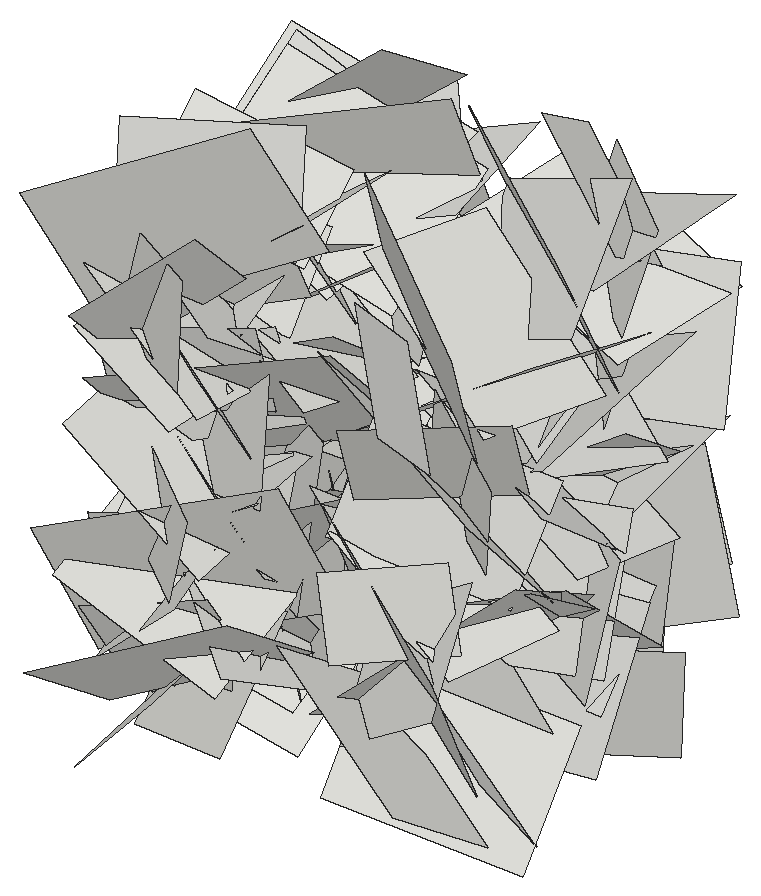
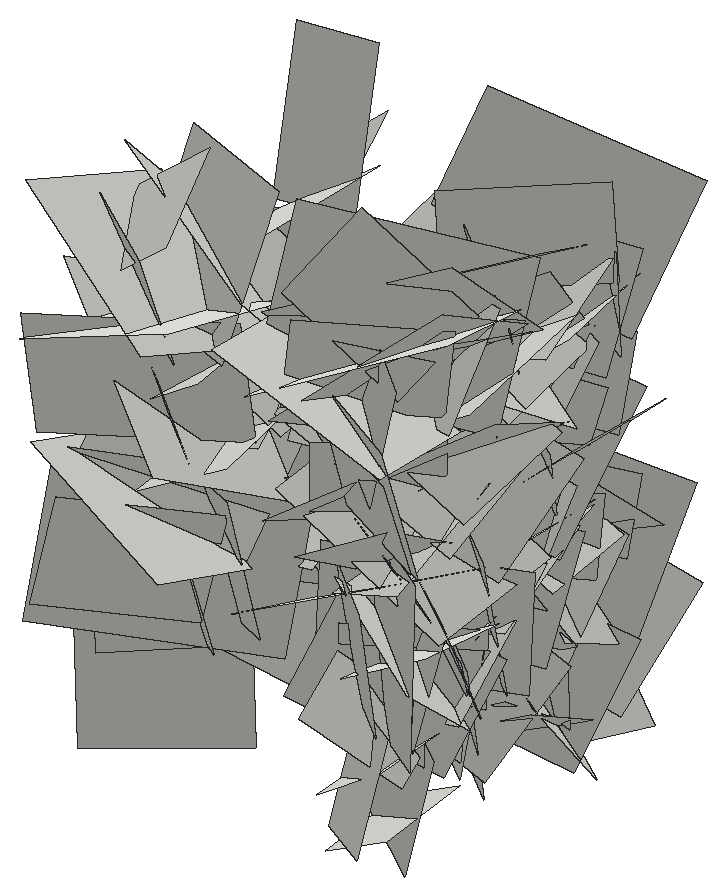
# SketchUp Ruby script. Lengths in inches.
U = 1.inch
M = Sketchup.active_model
def pt(a) = Geom::Point3d.new(a.map { |v| v * U })
def face(e, loops, mat)
  f = e.add_face(loops[0].map { |a| pt(a) })
  loops[1..].each { |l| e.add_face(l.map { |a| pt(a) }).erase! }
  f.material = f.back_material = mat if mat
  f
end
# faces: each face lists its corners as indices into pts; further lists are holes
def faces(e, pts, list, mat = nil) = list.each { |f| face(e, (f[0].is_a?(Array) ? f : [f]).map { |l| l.map { |i| pts[i] } }, mat) }
# xy, xz, yz: faces in a plane at the given z, y or x. An outline is a flat list of corners, or four numbers for a rectangle; further outlines are holes
def ring(l) = l.size == 4 ? [[l[0], l[1]], [l[2], l[1]], [l[2], l[3]], [l[0], l[3]]] : l.each_slice(2).to_a
def flat(e, list, mat, &to3) = list.each { |f| face(e, (f[0].is_a?(Array) ? f : [f]).map { |l| ring(l).map { |u, v| to3.(u, v) } }, mat) }
def xy(e, z, list, mat = nil) = flat(e, list, mat) { |x, y| [x, y, z] }
def xz(e, y, list, mat = nil) = flat(e, list, mat) { |x, z| [x, y, z] }
def yz(e, x, list, mat = nil) = flat(e, list, mat) { |y, z| [x, y, z] }
def lines(e, pts, list) = list.each { |a, b| e.add_line(pt(pts[a]), pt(pts[b])) }
# prism: a flat outline (further loops are holes) pulled along v
def prism(e, loops, v, mat = nil)
  f = face(e, loops, mat); d = Geom::Vector3d.new(v.map { |x| x * U })
  f.pushpull(f.normal.samedirection?(d) ? d.length : -d.length)
end
def box(e, o, s, mat = nil) = prism(e, [[o, [o[0] + s[0], o[1], o[2]], [o[0] + s[0], o[1] + s[1], o[2]], [o[0], o[1] + s[1], o[2]]]], [0, 0, s[2]], mat)
def at(x, y, z, deg = 0) = Geom::Transformation.translation(pt([x, y, z])) * Geom::Transformation.rotation(ORIGIN, Z_AXIS, deg.degrees)
def axes(o, x, y, z) = Geom::Transformation.new([*x, 0, *y, 0, *z, 0, *pt(o).to_a, 1])
def part(name) = M.definitions.add(name)
# library, detail: a bought-in or finely detailed component or shape, given as its bounding box
def library(name, o, s) = part(name).tap { |d| box(d.entities, o, s) }
def detail(e, o, s) = box(e.add_group.entities, o, s)
def put(e, d, t, mat = nil) = e.add_instance(d, t).tap { |i| i.material = mat if mat }
def group(e, t, mat = nil) = e.add_group.tap { |g| g.transformation = t; g.material = mat if mat }.entities
root = M.entities
c1 = part("Component\#6")
p = [[0.01,0,0],[0,3.24,4.54],[4.32,3.24,4.54],[4.33,0,0]]
faces(c1.entities,p,[[0,1,2,3]])
put(root,c1,axes([28.31,153.18,27.99],[0.08911,-1.01671,-0.11332],[0.1646,-0.0997,1.00972],[-1.07181,-0.09984,0.14565]))
put(root,c1,axes([24.34,160.42,26.72],[-0.04031,-0.6417,-0.5437],[0.04231,-0.54502,0.64047],[0.89052,-0.00315,-0.05504]))
put(root,c1,axes([28.31,152.86,32.22],[0.07765,-0.95123,0.12327],[0.10469,0.13045,0.94796],[-1.01133,-0.05954,0.1076]))
put(root,c1,axes([28.31,152.23,36.27],[-0.17612,0.33723,0.58016],[0.03508,0.60107,-0.33991],[-0.71045,-0.05392,-0.16061]))
put(root,c1,axes([24.34,156.02,27.27],[0.01737,0.78195,0.05447],[0.0729,0.05284,-0.77921],[0.82768,-0.02106,0.06749]))
put(root,c1,axes([24.34,151.43,29.49],[-0.01376,0.93036,0.01045],[-0.09599,0.00914,-0.92605],[0.98156,0.01394,-0.09041]))
put(root,c1,axes([24.34,155.63,34.51],[-0.04715,-0.7148,-0.47013],[0.06325,-0.47221,0.71232],[0.90467,-0.00424,-0.0743]))
put(root,c1,axes([28.31,159.35,19.53],[-0.12506,-0.65018,0.20227],[0.00025,0.20525,0.65988],[-0.72178,0.11273,-0.03482]))
put(root,c1,axes([28.31,154.14,39.875],[0.07687,-0.17009,-0.90128],[0.07958,-0.89996,0.17589],[-0.96896,-0.0874,-0.05706]))
put(root,c1,axes([24.34,161.57,34.4],[-0.05292,-0.24359,-0.78611],[0.1523,-0.77804,0.23197],[0.85897,0.12294,-0.08956]))
put(root,c1,axes([24.34,150.44,37.52],[-0.01758,-0.03984,-0.83316],[0.08726,-0.82933,0.03802],[0.87984,0.08145,-0.02042]))
put(root,c1,axes([24.34,152.86,25.21],[0.07237,-0.84668,-0.40971],[-0.16913,-0.41526,0.83156],[0.98259,-0.00911,0.17331]))
put(root,c1,axes([24.34,151.53,22],[-0.08087,0.78957,0.40941],[0.10212,0.41583,-0.78401],[0.93722,0.02282,0.12075]))
put(root,c1,axes([24.34,158.82,28.52],[-0.0834,-0.34729,-0.88838],[0.00654,-0.89156,0.34799],[1.01106,-0.02288,-0.07553]))
put(root,c1,axes([28.31,156.05,22.34],[-0.04217,-0.56806,-0.37659],[-0.07293,-0.37196,0.56834],[-0.71876,0.07107,-0.03557]))
put(root,c1,axes([28.31,160.84,30.26],[-0.09118,-0.56201,-0.30691],[-0.0596,-0.30185,0.56849],[-0.67615,0.1024,-0.00872]))
put(root,c1,axes([24.34,154.61,36.92],[-0.07328,1.03426,0.55463],[-0.26621,0.52968,-1.01904],[1.21518,0.17841,-0.1898]))
put(root,c1,axes([28.31,159.76,21.63],[-0.09665,-0.666,0.12875],[0.03078,0.12595,0.67212],[-0.71837,0.095,0.01147]))
put(root,c1,axes([28.31,147.16,24.1],[0.03025,0.92414,0.23442],[0.23339,0.2218,-0.90118],[-0.98329,0.08108,-0.20669]))
put(root,c1,axes([24.34,157.73,31.39],[-0.13129,-0.92283,0.37392],[0.04334,0.37177,0.93107],[1.05456,-0.13017,0.00829]))
put(root,c1,axes([28.31,159.1875,20.3125],[0.01409,-0.35632,0.80543],[0.16766,0.79339,0.34838],[-0.91839,0.13938,0.07596]))
put(root,c1,axes([28.31,153.92,21.15],[0.0271,-0.2919,0.8704],[0.20523,0.85287,0.28034],[-0.95124,0.17569,0.08528]))
put(root,c1,axes([28.31,149.63,26.39],[0.05575,0.3601,-0.58557],[-0.15834,-0.56726,-0.36226],[-0.71127,0.15451,0.03475]))
put(root,c1,axes([28.31,150.69,21.46],[0.08617,-0.06424,0.73191],[-0.1147,0.7273,0.07585],[-0.77031,-0.11548,0.07058]))
put(root,c1,axes([24.34,152.31,24.83],[0.14132,0.38772,0.61473],[0.11706,0.60692,-0.40674],[0.76145,-0.16526,-0.05156]))
put(root,c1,axes([24.34,150.4,30.92],[0.04252,-0.27759,0.76161],[0.13298,0.75548,0.26875],[0.84891,-0.10444,-0.08025]))
put(root,c1,axes([28.31,156.49,28.09],[-0.01227,0.36562,0.53928],[-0.0952,0.53332,-0.36351],[-0.68404,-0.08079,0.04092]))
put(root,c1,axes([24.34,150.56,37.37],[0.01495,0.72639,-0.4873],[0.06872,-0.48689,-0.7239],[0.92463,0.02444,0.06168]))
put(root,c1,axes([28.31,156.34,37.48],[0.20366,-0.78098,-0.33642],[-0.07649,-0.35863,0.79133],[-0.89812,-0.14656,-0.14368]))
put(root,c1,axes([24.34,156.72,22.08],[-0.00521,-0.94479,0.50901],[-0.17637,0.50353,0.93301],[1.12382,0.07464,0.14878]))
put(root,c1,axes([28.31,158.75,26.14],[-0.12859,0.59437,-0.23179],[0.06253,-0.22448,-0.60651],[-0.67335,-0.13435,-0.01206]))
put(root,c1,axes([24.34,154.45,36.57],[0.07713,0.81709,0.22722],[0.03645,0.22503,-0.82021],[0.89825,-0.07929,0.01378]))
put(root,c1,axes([28.31,149.71,29.1],[-0.04042,0.22115,-0.567],[-0.10046,-0.56334,-0.21335],[-0.63725,0.07479,0.0696]))
put(root,c1,axes([28.31,153.82,25.23],[-0.04726,-0.11023,0.59197],[-0.093,0.58845,0.10297],[-0.63147,-0.07841,-0.05947]))
put(root,c1,axes([24.34,150.92,33.45],[-0.01124,-0.40239,0.85237],[0.02564,0.85203,0.40253],[0.99881,-0.0264,-0.00074]))
put(root,c1,axes([24.34,152.27,30.34],[0.04267,0.47891,-0.74389],[0.05776,-0.74459,-0.47642],[0.93603,0.02411,0.06331]))
put(root,c1,axes([24.34,153.79,24.7],[-0.00565,-0.43188,0.90191],[-0.04751,0.90112,0.43124],[1.05892,0.03812,0.02416]))
put(root,c1,axes([24.34,160.9375,37.33],[0.13153,0.12633,-0.90974],[-0.10231,-0.91113,-0.13969],[0.96819,-0.11344,0.10882]))
put(root,c1,axes([28.31,155.3,36.05],[0.02231,-0.46484,-0.62566],[0.10069,-0.6197,0.4636],[-0.82005,-0.08874,0.0399]))
put(root,c1,axes([24.34,155.99,38.05],[0.0315,0.52335,-0.79271],[-0.01447,-0.79278,-0.52391],[1.00678,-0.02777,0.01727]))
put(root,c1,axes([28.31,150.81,32.67],[0.03105,-0.70657,0.01303],[-0.00041,0.01303,0.70717],[-0.74909,-0.02929,0.00015]))
put(root,c1,axes([24.34,158.65,23.12],[-0.03,-0.65446,0.65644],[0.11713,0.64968,0.65248],[0.97555,-0.09812,-0.05816]))
put(root,c1,axes([28.31,151.89,27.92],[-0.07457,-0.37507,-0.49968],[0.035,-0.50437,0.37394],[-0.66135,0.0156,0.07613]))
put(root,c1,axes([28.31,158.01,30.39],[-0.08038,-0.60995,0.00551],[0.02253,0.00291,0.6143],[-0.64618,0.07598,0.02073]))
put(root,c1,axes([28.31,153.52,29.46],[0.08102,0.00764,-0.81457],[0.10707,-0.81193,0.00187],[-0.85682,-0.10074,-0.07679]))
put(root,c1,axes([24.34,152.65,32.7],[-0.31384,1.21799,0.62272],[-0.13011,0.61092,-1.25326],[1.44417,0.31973,0.02242]))
put(root,c1,axes([24.34,149.65,34.23],[-0.2234,-0.54463,1.08834],[-0.02633,1.10624,0.54877],[1.28976,-0.07175,0.19972]))
put(root,c1,axes([28.31,152.7,33.94],[0.15183,0.13661,-0.74127],[-0.04087,-0.75222,-0.14607],[-0.79793,0.06452,-0.13357]))
put(root,c1,axes([28.31,158.73,27.09],[0.13155,-0.14233,-0.74779],[0.00006,-0.75766,0.14422],[-0.80689,-0.02326,-0.12191]))
put(root,c1,axes([24.34,158.66,27.8],[0.19419,0.10037,-0.91545],[-0.10975,-0.92523,-0.12216],[0.97001,-0.12478,0.16945]))
put(root,c1,axes([28.31,156.65,23.33],[-0.01341,0.01203,0.69899],[0.10657,0.69187,-0.01009],[-0.73333,0.10033,-0.01425]))
put(root,c1,axes([24.34,154.96,37.56],[-0.27688,1.1515,0.31839],[0.11464,0.34737,-1.16756],[1.26119,0.22122,0.17603]))
put(root,c1,axes([24.34,152.42,20.54],[-0.05004,-0.6691,0.77955],[0.05919,0.77755,0.67076],[1.08735,-0.07312,-0.00064]))
put(root,c1,axes([28.31,161,38.46],[0.19651,-0.13504,-0.81499],[0.03185,-0.8336,0.14496],[-0.87508,-0.06067,-0.17773]))
put(root,c1,axes([24.34,159.15,23.91],[0.14407,0.13595,-0.90237],[-0.02833,-0.91134,-0.14133],[0.9669,-0.04696,0.13032]))
put(root,c1,axes([24.34,151.25,34.8],[0.16779,0.3958,-0.75565],[0.05631,-0.77163,-0.39305],[0.90246,-0.02545,0.16502]))
put(root,c1,axes([28.31,158.03,24.73],[0.19324,-0.05037,0.89121],[0.15909,0.89838,0.02008],[-0.93272,0.1428,0.18806]))
put(root,c1,axes([24.34,154.4,23.625],[-0.0407,-0.65785,-0.83395],[0.03781,-0.83482,0.65689],[1.12528,0.00426,-0.05223]))
put(root,c1,axes([28.31,157.59,40.82],[0.16311,0.68993,-0.43022],[0.09586,-0.44966,-0.68876],[-0.85651,0.08106,-0.15901]))
put(root,c1,axes([24.34,154.59,24.16],[-0.1724,0.15274,1.09758],[0.17194,1.10067,-0.12914],[1.16199,-0.14021,0.18195]))
put(root,c1,axes([24.34,152.14,28.92],[0.00837,0.82237,-0.50147],[0.16225,-0.49618,-0.8113],[1.00803,0.07304,0.13474]))
put(root,c1,axes([28.31,149.08,38.35],[-0.0057,0.54335,-0.52891],[0.23788,-0.50408,-0.52014],[-0.76776,-0.16022,-0.15723]))
put(root,c1,axes([28.31,157.4,31.875],[0.05779,-0.51798,-0.36432],[0.0587,-0.36037,0.52065],[-0.6687,-0.0764,0.01422]))
put(root,c1,axes([24.34,156.45,32.24],[0.14884,0.843,-0.57449],[-0.06248,-0.57223,-0.85409],[1.07954,-0.14935,0.02978]))
put(root,c1,axes([28.31,160.09,33.87],[0.13785,-0.16653,-0.67513],[0.04892,-0.68326,0.17743],[-0.73546,-0.07666,-0.11474]))
put(root,c1,axes([24.34,156.02,28.65],[-0.0619,-0.85924,0.62732],[0.17366,0.61351,0.85557],[1.11425,-0.14335,-0.09849]))
put(root,c1,axes([28.31,147.9,27.03],[0.12769,0.03013,0.63893],[0.01482,0.64988,-0.03329],[-0.67785,0.01989,0.11963]))
put(root,c1,axes([24.34,156.69,29.48],[-0.02364,1.01192,0.31394],[0.16386,0.31376,-1.00035],[1.11105,-0.02474,0.15421]))
put(root,c1,axes([24.34,161.68,35.57],[-0.09547,-0.29138,-1.10436],[0.14499,-1.10257,0.27976],[1.20197,0.10985,-0.12146]))
put(root,c1,axes([24.34,147.58,26.68],[0.22766,0.71104,0.67114],[-0.02672,0.69094,-0.72395],[1.03608,-0.13842,-0.16614]))
put(root,c1,axes([24.34,153.43,27.14],[0.15407,-0.97446,-0.01303],[0.08051,-0.00181,0.98239],[1.02988,0.14592,-0.07485]))
put(root,c1,axes([24.34,158.93,27.77],[-0.0679,-1.16178,0.21088],[0.08573,0.20637,1.16154],[1.24867,-0.07734,-0.06828]))
put(root,c1,axes([24.34,160.05,30.35],[-0.12426,0.20575,-1.35522],[-0.11745,-1.35714,-0.19646],[1.44825,-0.0924,-0.13221]))
put(root,c1,axes([24.34,157.84,26.69],[0.16666,-0.37984,-0.88441],[0.10341,-0.88523,0.39754],[1.01503,0.15255,0.10471]))
put(root,c1,axes([24.34,153.58,31.99],[0.17505,-0.32324,-0.90395],[0.10086,-0.9072,0.34179],[1.0126,0.14624,0.12223]))
put(root,c1,axes([24.34,151.45,29.33],[0.11063,1.17252,-0.59491],[-0.28501,-0.56514,-1.16101],[1.36425,-0.21315,-0.19431]))
put(root,c1,axes([24.34,155.57,33.875],[0.13701,-1.11756,0.11199],[-0.07264,0.10468,1.12363],[1.18833,0.13525,0.05577]))
put(root,c1,axes([24.34,156.79,29.67],[0.01777,-0.29003,-1.18393],[-0.05362,-1.18318,0.28913],[1.29096,-0.04516,0.0283]))
put(root,c1,axes([24.34,158.37,30.5],[0.12568,-1.12455,0.31778],[-0.06348,0.31314,1.13049],[1.23707,0.13032,0.02572]))
put(root,c1,axes([24.34,152.25,36.24],[-0.0137,1.21221,-0.26433],[0.01965,-0.26413,-1.21218],[1.31499,0.01657,0.01536]))
put(root,c1,axes([24.34,150.2,21.48],[0.03659,-0.96074,0.6365],[0.08804,0.6372,0.9573],[1.21843,-0.01719,-0.08829]))
put(root,c1,axes([24.34,149.67,23.37],[-0.09539,-0.59855,1.14231],[0.08783,1.14003,0.60389],[1.36418,-0.11525,0.041]))
put(root,c1,axes([24.34,153.92,36.42],[0.14295,0.82362,0.79821],[0.11339,0.79118,-0.83443],[1.21047,-0.17138,-0.0161]))
put(root,c1,axes([24.34,156.14,33.68],[0.06217,-0.55405,1.15944],[0.03014,1.16092,0.55332],[1.36179,-0.0004,-0.06518]))
put(root,c1,axes([24.34,157.5625,26.25],[0.15158,-0.38022,-1.22414],[-0.0526,-1.23246,0.37701],[1.35773,-0.0053,0.15127]))
put(root,c1,axes([24.34,161.74,34.71],[0.1652,-1.10091,-0.16395],[0.26327,-0.12698,1.08875],[1.15009,0.1872,-0.22568]))
put(root,c1,axes([24.34,153.73,28.3],[-0.01858,0.99462,-0.84655],[0.29457,-0.8244,-0.97435],[1.35277,0.19318,0.20054]))
put(root,c1,axes([24.34,153.125,28.17],[-0.03085,-0.9293,0.97672],[0.26234,0.95667,0.91759],[1.40479,-0.19906,-0.14991]))
put(root,c1,axes([24.34,153.14,23.91],[0.18,-1.08552,0.79109],[0.08355,0.80406,1.08641],[1.42134,0.0902,-0.16405]))
put(root,c1,axes([38.11,153.14,23.91],[-0.18,-1.08552,0.79109],[-0.08355,0.80406,1.08641],[-1.42134,0.0902,-0.16405]))
put(root,c1,axes([38.11,153.125,28.17],[0.03085,-0.9293,0.97672],[-0.26234,0.95667,0.91759],[-1.40479,-0.19906,-0.14991]))
put(root,c1,axes([38.11,153.73,28.3],[0.01858,0.99462,-0.84655],[-0.29457,-0.8244,-0.97435],[-1.35277,0.19318,0.20054]))
put(root,c1,axes([38.11,161.74,34.71],[-0.1652,-1.10091,-0.16395],[-0.26327,-0.12698,1.08875],[-1.15009,0.1872,-0.22568]))
put(root,c1,axes([38.11,157.5625,26.25],[-0.15158,-0.38022,-1.22414],[0.0526,-1.23246,0.37701],[-1.35773,-0.0053,0.15127]))
put(root,c1,axes([38.11,156.14,33.68],[-0.06217,-0.55405,1.15944],[-0.03014,1.16092,0.55332],[-1.36179,-0.0004,-0.06518]))
put(root,c1,axes([38.11,153.92,36.42],[-0.14295,0.82362,0.79821],[-0.11339,0.79118,-0.83443],[-1.21047,-0.17138,-0.0161]))
put(root,c1,axes([38.11,149.67,23.37],[0.09539,-0.59855,1.14231],[-0.08783,1.14003,0.60389],[-1.36418,-0.11525,0.041]))
put(root,c1,axes([38.11,150.2,21.48],[-0.03659,-0.96074,0.6365],[-0.08804,0.6372,0.9573],[-1.21843,-0.01719,-0.08829]))
put(root,c1,axes([38.11,152.25,36.24],[0.0137,1.21221,-0.26433],[-0.01965,-0.26413,-1.21218],[-1.31499,0.01657,0.01536]))
put(root,c1,axes([38.11,158.37,30.5],[-0.12568,-1.12455,0.31778],[0.06348,0.31314,1.13049],[-1.23707,0.13032,0.02572]))
put(root,c1,axes([38.11,156.79,29.67],[-0.01777,-0.29003,-1.18393],[0.05362,-1.18318,0.28913],[-1.29096,-0.04516,0.0283]))
put(root,c1,axes([38.11,155.57,33.875],[-0.13701,-1.11756,0.11199],[0.07264,0.10468,1.12363],[-1.18833,0.13525,0.05577]))
put(root,c1,axes([38.11,151.45,29.33],[-0.11063,1.17252,-0.59491],[0.28501,-0.56514,-1.16101],[-1.36425,-0.21315,-0.19431]))
put(root,c1,axes([38.11,153.58,31.99],[-0.17505,-0.32324,-0.90395],[-0.10086,-0.9072,0.34179],[-1.0126,0.14624,0.12223]))
put(root,c1,axes([38.11,157.84,26.69],[-0.16666,-0.37984,-0.88441],[-0.10341,-0.88523,0.39754],[-1.01503,0.15255,0.10471]))
put(root,c1,axes([38.11,160.05,30.35],[0.12426,0.20575,-1.35522],[0.11745,-1.35714,-0.19646],[-1.44825,-0.0924,-0.13221]))
put(root,c1,axes([38.11,158.93,27.77],[0.0679,-1.16178,0.21088],[-0.08573,0.20637,1.16154],[-1.24867,-0.07734,-0.06828]))
put(root,c1,axes([38.11,153.43,27.14],[-0.15407,-0.97446,-0.01303],[-0.08051,-0.00181,0.98239],[-1.02988,0.14592,-0.07485]))
put(root,c1,axes([38.11,147.58,26.68],[-0.22766,0.71104,0.67114],[0.02672,0.69094,-0.72395],[-1.03608,-0.13842,-0.16614]))
put(root,c1,axes([38.11,161.68,35.57],[0.09547,-0.29138,-1.10436],[-0.14499,-1.10257,0.27976],[-1.20197,0.10985,-0.12146]))
put(root,c1,axes([38.11,156.69,29.48],[0.02364,1.01192,0.31394],[-0.16386,0.31376,-1.00035],[-1.11105,-0.02474,0.15421]))
put(root,c1,axes([34.14,147.9,27.03],[-0.12769,0.03013,0.63893],[-0.01482,0.64988,-0.03329],[0.67785,0.01989,0.11963]))
put(root,c1,axes([38.11,156.02,28.65],[0.0619,-0.85924,0.62732],[-0.17366,0.61351,0.85557],[-1.11425,-0.14335,-0.09849]))
put(root,c1,axes([34.14,160.09,33.87],[-0.13785,-0.16653,-0.67513],[-0.04892,-0.68326,0.17743],[0.73546,-0.07666,-0.11474]))
put(root,c1,axes([38.11,156.45,32.24],[-0.14884,0.843,-0.57449],[0.06248,-0.57223,-0.85409],[-1.07954,-0.14935,0.02978]))
put(root,c1,axes([34.14,157.4,31.875],[-0.05779,-0.51798,-0.36432],[-0.0587,-0.36037,0.52065],[0.6687,-0.0764,0.01422]))
put(root,c1,axes([34.14,149.08,38.35],[0.0057,0.54335,-0.52891],[-0.23788,-0.50408,-0.52014],[0.76776,-0.16022,-0.15723]))
put(root,c1,axes([38.11,152.14,28.92],[-0.00837,0.82237,-0.50147],[-0.16225,-0.49618,-0.8113],[-1.00803,0.07304,0.13474]))
put(root,c1,axes([38.11,154.59,24.16],[0.1724,0.15274,1.09758],[-0.17194,1.10067,-0.12914],[-1.16199,-0.14021,0.18195]))
put(root,c1,axes([34.14,157.59,40.82],[-0.16311,0.68993,-0.43022],[-0.09586,-0.44966,-0.68876],[0.85651,0.08106,-0.15901]))
put(root,c1,axes([38.11,154.4,23.625],[0.0407,-0.65785,-0.83395],[-0.03781,-0.83482,0.65689],[-1.12528,0.00426,-0.05223]))
put(root,c1,axes([34.14,158.03,24.73],[-0.19324,-0.05037,0.89121],[-0.15909,0.89838,0.02008],[0.93272,0.1428,0.18806]))
put(root,c1,axes([38.11,151.25,34.8],[-0.16779,0.3958,-0.75565],[-0.05631,-0.77163,-0.39305],[-0.90246,-0.02545,0.16502]))
put(root,c1,axes([38.11,159.15,23.91],[-0.14407,0.13595,-0.90237],[0.02833,-0.91134,-0.14133],[-0.9669,-0.04696,0.13032]))
put(root,c1,axes([34.14,161,38.46],[-0.19651,-0.13504,-0.81499],[-0.03185,-0.8336,0.14496],[0.87508,-0.06067,-0.17773]))
put(root,c1,axes([38.11,152.42,20.54],[0.05004,-0.6691,0.77955],[-0.05919,0.77755,0.67076],[-1.08735,-0.07312,-0.00064]))
put(root,c1,axes([38.11,154.96,37.56],[0.27688,1.1515,0.31839],[-0.11464,0.34737,-1.16756],[-1.26119,0.22122,0.17603]))
put(root,c1,axes([34.14,156.65,23.33],[0.01341,0.01203,0.69899],[-0.10657,0.69187,-0.01009],[0.73333,0.10033,-0.01425]))
put(root,c1,axes([38.11,158.66,27.8],[-0.19419,0.10037,-0.91545],[0.10975,-0.92523,-0.12216],[-0.97001,-0.12478,0.16945]))
put(root,c1,axes([34.14,158.73,27.09],[-0.13155,-0.14233,-0.74779],[-0.00006,-0.75766,0.14422],[0.80689,-0.02326,-0.12191]))
put(root,c1,axes([34.14,152.7,33.94],[-0.15183,0.13661,-0.74127],[0.04087,-0.75222,-0.14607],[0.79793,0.06452,-0.13357]))
put(root,c1,axes([38.11,149.65,34.23],[0.2234,-0.54463,1.08834],[0.02633,1.10624,0.54877],[-1.28976,-0.07175,0.19972]))
put(root,c1,axes([38.11,152.65,32.7],[0.31384,1.21799,0.62272],[0.13011,0.61092,-1.25326],[-1.44417,0.31973,0.02242]))
